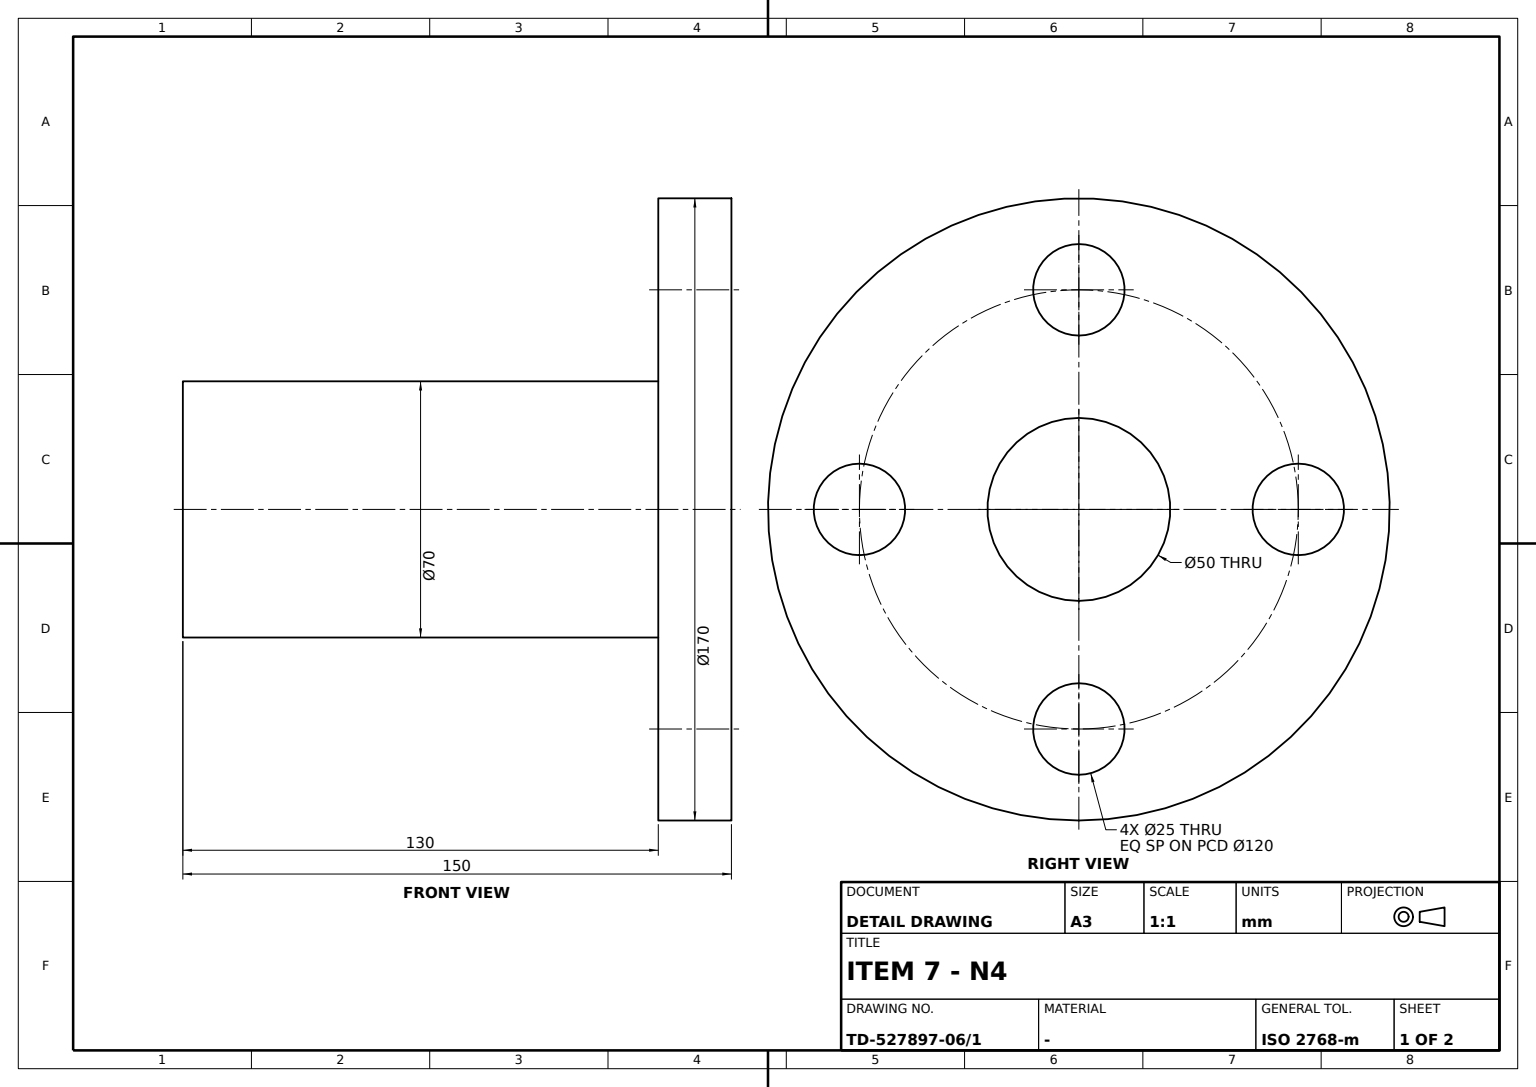
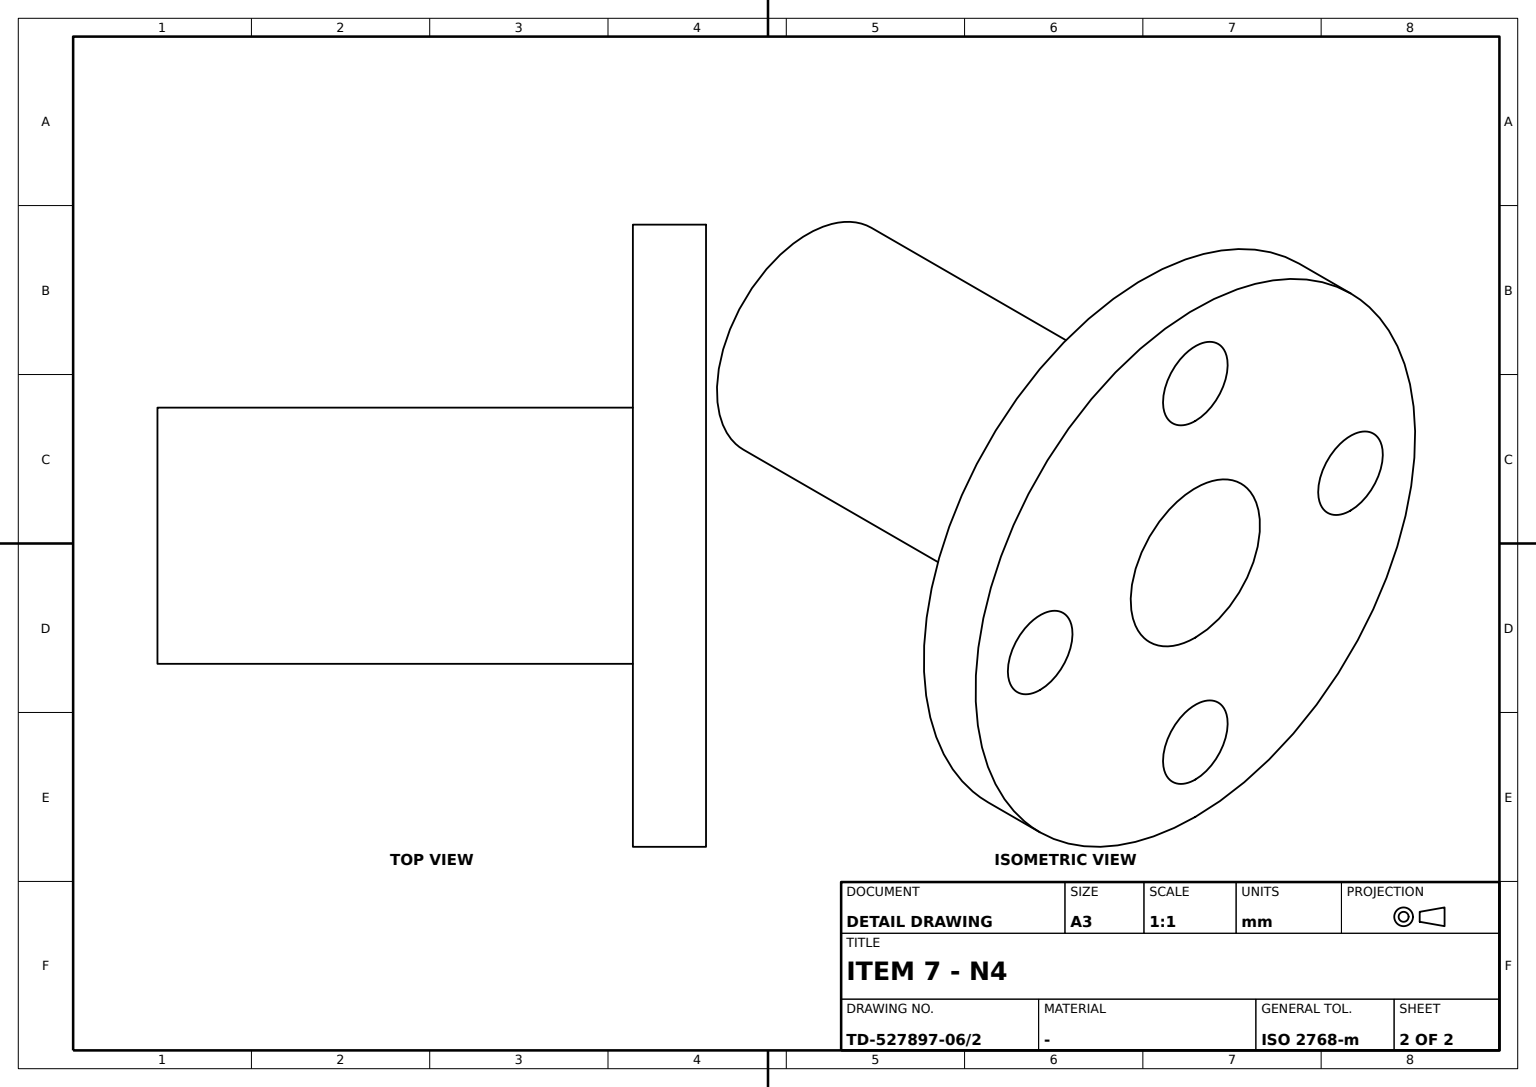
ISO-10303-21;
HEADER;
FILE_DESCRIPTION((''),'2;1');
FILE_NAME('','',(''),(''),'','','');
FILE_SCHEMA(('AUTOMOTIVE_DESIGN'));
ENDSEC;
DATA;
#1=APPLICATION_CONTEXT('');
#2=PRODUCT_CONTEXT('',#1,'mechanical');
#3=PRODUCT('','','',(#2));
#4=PRODUCT_DEFINITION_FORMATION('','',#3);
#5=PRODUCT_DEFINITION_CONTEXT('',#1,'design');
#6=PRODUCT_DEFINITION('','',#4,#5);
#7=PRODUCT_DEFINITION_SHAPE('','',#6);
#8=(LENGTH_UNIT()NAMED_UNIT(*)SI_UNIT(.MILLI.,.METRE.));
#9=(NAMED_UNIT(*)PLANE_ANGLE_UNIT()SI_UNIT($,.RADIAN.));
#10=(NAMED_UNIT(*)SI_UNIT($,.STERADIAN.)SOLID_ANGLE_UNIT());
#11=UNCERTAINTY_MEASURE_WITH_UNIT(LENGTH_MEASURE(0.005),#8,'distance_accuracy_value','');
#12=(GEOMETRIC_REPRESENTATION_CONTEXT(3)GLOBAL_UNCERTAINTY_ASSIGNED_CONTEXT((#11))GLOBAL_UNIT_ASSIGNED_CONTEXT((#8,#9,#10))REPRESENTATION_CONTEXT('',''));
#13=CARTESIAN_POINT('',(1202.5,1250.,2650.));
#14=VERTEX_POINT('',#13);
#15=CARTESIAN_POINT('',(1190.,1250.,2650.));
#16=DIRECTION('',(0.,0.,1.));
#17=DIRECTION('',(1.,0.,0.));
#18=AXIS2_PLACEMENT_3D('',#15,#16,#17);
#19=CIRCLE('',#18,12.5);
#20=EDGE_CURVE('',#14,#14,#19,.T.);
#21=ORIENTED_EDGE('',*,*,#20,.T.);
#22=EDGE_LOOP('',(#21));
#23=FACE_BOUND('',#22,.T.);
#24=CARTESIAN_POINT('',(1202.5,1250.,2630.));
#25=VERTEX_POINT('',#24);
#26=CARTESIAN_POINT('',(1190.,1250.,2630.));
#27=AXIS2_PLACEMENT_3D('',#26,#16,#17);
#28=CIRCLE('',#27,12.5);
#29=EDGE_CURVE('',#25,#25,#28,.T.);
#30=ORIENTED_EDGE('',*,*,#29,.F.);
#31=EDGE_LOOP('',(#30));
#32=FACE_BOUND('',#31,.T.);
#33=CARTESIAN_POINT('',(1190.,1250.,2640.));
#34=AXIS2_PLACEMENT_3D('',#33,#16,#17);
#35=CYLINDRICAL_SURFACE('',#34,12.5);
#36=ADVANCED_FACE('',(#23,#32),#35,.F.);
#37=CARTESIAN_POINT('',(1262.5,1190.,2630.));
#38=VERTEX_POINT('',#37);
#39=CARTESIAN_POINT('',(1250.,1190.,2630.));
#40=AXIS2_PLACEMENT_3D('',#39,#16,#17);
#41=CIRCLE('',#40,12.5);
#42=EDGE_CURVE('',#38,#38,#41,.T.);
#43=ORIENTED_EDGE('',*,*,#42,.T.);
#44=EDGE_LOOP('',(#43));
#45=FACE_BOUND('',#44,.T.);
#46=CARTESIAN_POINT('',(1335.,1250.,2630.));
#47=VERTEX_POINT('',#46);
#48=CARTESIAN_POINT('',(1250.,1250.,2630.));
#49=AXIS2_PLACEMENT_3D('',#48,#16,#17);
#50=CIRCLE('',#49,85.);
#51=EDGE_CURVE('',#47,#47,#50,.T.);
#52=ORIENTED_EDGE('',*,*,#51,.F.);
#53=EDGE_LOOP('',(#52));
#54=FACE_BOUND('',#53,.T.);
#55=CARTESIAN_POINT('',(1322.5,1250.,2630.));
#56=VERTEX_POINT('',#55);
#57=CARTESIAN_POINT('',(1310.,1250.,2630.));
#58=AXIS2_PLACEMENT_3D('',#57,#16,#17);
#59=CIRCLE('',#58,12.5);
#60=EDGE_CURVE('',#56,#56,#59,.T.);
#61=ORIENTED_EDGE('',*,*,#60,.T.);
#62=EDGE_LOOP('',(#61));
#63=FACE_BOUND('',#62,.T.);
#64=ORIENTED_EDGE('',*,*,#29,.T.);
#65=EDGE_LOOP('',(#64));
#66=FACE_BOUND('',#65,.T.);
#67=CARTESIAN_POINT('',(1262.5,1310.,2630.));
#68=VERTEX_POINT('',#67);
#69=CARTESIAN_POINT('',(1250.,1310.,2630.));
#70=AXIS2_PLACEMENT_3D('',#69,#16,#17);
#71=CIRCLE('',#70,12.5);
#72=EDGE_CURVE('',#68,#68,#71,.T.);
#73=ORIENTED_EDGE('',*,*,#72,.T.);
#74=EDGE_LOOP('',(#73));
#75=FACE_BOUND('',#74,.T.);
#76=CARTESIAN_POINT('',(1285.,1250.,2630.));
#77=VERTEX_POINT('',#76);
#78=CIRCLE('',#49,35.);
#79=EDGE_CURVE('',#77,#77,#78,.T.);
#80=ORIENTED_EDGE('',*,*,#79,.T.);
#81=EDGE_LOOP('',(#80));
#82=FACE_BOUND('',#81,.T.);
#83=CARTESIAN_POINT('',(0.,0.,2630.));
#84=AXIS2_PLACEMENT_3D('',#83,#16,#17);
#85=PLANE('',#84);
#86=ADVANCED_FACE('',(#45,#54,#63,#66,#75,#82),#85,.F.);
#87=ORIENTED_EDGE('',*,*,#51,.T.);
#88=EDGE_LOOP('',(#87));
#89=FACE_BOUND('',#88,.T.);
#90=CARTESIAN_POINT('',(1335.,1250.,2650.));
#91=VERTEX_POINT('',#90);
#92=CARTESIAN_POINT('',(1250.,1250.,2650.));
#93=AXIS2_PLACEMENT_3D('',#92,#16,#17);
#94=CIRCLE('',#93,85.);
#95=EDGE_CURVE('',#91,#91,#94,.T.);
#96=ORIENTED_EDGE('',*,*,#95,.F.);
#97=EDGE_LOOP('',(#96));
#98=FACE_BOUND('',#97,.T.);
#99=CARTESIAN_POINT('',(1250.,1250.,2640.));
#100=AXIS2_PLACEMENT_3D('',#99,#16,#17);
#101=CYLINDRICAL_SURFACE('',#100,85.);
#102=ADVANCED_FACE('',(#89,#98),#101,.T.);
#103=ORIENTED_EDGE('',*,*,#72,.F.);
#104=EDGE_LOOP('',(#103));
#105=FACE_BOUND('',#104,.T.);
#106=CARTESIAN_POINT('',(1262.5,1310.,2650.));
#107=VERTEX_POINT('',#106);
#108=CARTESIAN_POINT('',(1250.,1310.,2650.));
#109=AXIS2_PLACEMENT_3D('',#108,#16,#17);
#110=CIRCLE('',#109,12.5);
#111=EDGE_CURVE('',#107,#107,#110,.T.);
#112=ORIENTED_EDGE('',*,*,#111,.T.);
#113=EDGE_LOOP('',(#112));
#114=FACE_BOUND('',#113,.T.);
#115=CARTESIAN_POINT('',(1250.,1310.,2640.));
#116=AXIS2_PLACEMENT_3D('',#115,#16,#17);
#117=CYLINDRICAL_SURFACE('',#116,12.5);
#118=ADVANCED_FACE('',(#105,#114),#117,.F.);
#119=CARTESIAN_POINT('',(1275.,1250.,2500.));
#120=VERTEX_POINT('',#119);
#121=CARTESIAN_POINT('',(1250.,1250.,2500.));
#122=AXIS2_PLACEMENT_3D('',#121,#16,#17);
#123=CIRCLE('',#122,25.);
#124=EDGE_CURVE('',#120,#120,#123,.T.);
#125=ORIENTED_EDGE('',*,*,#124,.F.);
#126=EDGE_LOOP('',(#125));
#127=FACE_BOUND('',#126,.T.);
#128=CARTESIAN_POINT('',(1275.,1250.,2650.));
#129=VERTEX_POINT('',#128);
#130=CIRCLE('',#93,25.);
#131=EDGE_CURVE('',#129,#129,#130,.T.);
#132=ORIENTED_EDGE('',*,*,#131,.T.);
#133=EDGE_LOOP('',(#132));
#134=FACE_BOUND('',#133,.T.);
#135=CARTESIAN_POINT('',(1250.,1250.,2575.));
#136=AXIS2_PLACEMENT_3D('',#135,#16,#17);
#137=CYLINDRICAL_SURFACE('',#136,25.);
#138=ADVANCED_FACE('',(#127,#134),#137,.F.);
#139=ORIENTED_EDGE('',*,*,#79,.F.);
#140=EDGE_LOOP('',(#139));
#141=FACE_BOUND('',#140,.T.);
#142=CARTESIAN_POINT('',(1285.,1250.,2500.));
#143=VERTEX_POINT('',#142);
#144=CIRCLE('',#122,35.);
#145=EDGE_CURVE('',#143,#143,#144,.T.);
#146=ORIENTED_EDGE('',*,*,#145,.T.);
#147=EDGE_LOOP('',(#146));
#148=FACE_BOUND('',#147,.T.);
#149=CYLINDRICAL_SURFACE('',#136,35.);
#150=ADVANCED_FACE('',(#141,#148),#149,.T.);
#151=ORIENTED_EDGE('',*,*,#20,.F.);
#152=EDGE_LOOP('',(#151));
#153=FACE_BOUND('',#152,.T.);
#154=CARTESIAN_POINT('',(1262.5,1190.,2650.));
#155=VERTEX_POINT('',#154);
#156=CARTESIAN_POINT('',(1250.,1190.,2650.));
#157=AXIS2_PLACEMENT_3D('',#156,#16,#17);
#158=CIRCLE('',#157,12.5);
#159=EDGE_CURVE('',#155,#155,#158,.T.);
#160=ORIENTED_EDGE('',*,*,#159,.F.);
#161=EDGE_LOOP('',(#160));
#162=FACE_BOUND('',#161,.T.);
#163=ORIENTED_EDGE('',*,*,#131,.F.);
#164=EDGE_LOOP('',(#163));
#165=FACE_BOUND('',#164,.T.);
#166=ORIENTED_EDGE('',*,*,#111,.F.);
#167=EDGE_LOOP('',(#166));
#168=FACE_BOUND('',#167,.T.);
#169=CARTESIAN_POINT('',(1322.5,1250.,2650.));
#170=VERTEX_POINT('',#169);
#171=CARTESIAN_POINT('',(1310.,1250.,2650.));
#172=AXIS2_PLACEMENT_3D('',#171,#16,#17);
#173=CIRCLE('',#172,12.5);
#174=EDGE_CURVE('',#170,#170,#173,.T.);
#175=ORIENTED_EDGE('',*,*,#174,.F.);
#176=EDGE_LOOP('',(#175));
#177=FACE_BOUND('',#176,.T.);
#178=ORIENTED_EDGE('',*,*,#95,.T.);
#179=EDGE_LOOP('',(#178));
#180=FACE_BOUND('',#179,.T.);
#181=CARTESIAN_POINT('',(0.,0.,2650.));
#182=AXIS2_PLACEMENT_3D('',#181,#16,#17);
#183=PLANE('',#182);
#184=ADVANCED_FACE('',(#153,#162,#165,#168,#177,#180),#183,.T.);
#185=ORIENTED_EDGE('',*,*,#60,.F.);
#186=EDGE_LOOP('',(#185));
#187=FACE_BOUND('',#186,.T.);
#188=ORIENTED_EDGE('',*,*,#174,.T.);
#189=EDGE_LOOP('',(#188));
#190=FACE_BOUND('',#189,.T.);
#191=CARTESIAN_POINT('',(1310.,1250.,2640.));
#192=AXIS2_PLACEMENT_3D('',#191,#16,#17);
#193=CYLINDRICAL_SURFACE('',#192,12.5);
#194=ADVANCED_FACE('',(#187,#190),#193,.F.);
#195=ORIENTED_EDGE('',*,*,#42,.F.);
#196=EDGE_LOOP('',(#195));
#197=FACE_BOUND('',#196,.T.);
#198=ORIENTED_EDGE('',*,*,#159,.T.);
#199=EDGE_LOOP('',(#198));
#200=FACE_BOUND('',#199,.T.);
#201=CARTESIAN_POINT('',(1250.,1190.,2640.));
#202=AXIS2_PLACEMENT_3D('',#201,#16,#17);
#203=CYLINDRICAL_SURFACE('',#202,12.5);
#204=ADVANCED_FACE('',(#197,#200),#203,.F.);
#205=ORIENTED_EDGE('',*,*,#145,.F.);
#206=EDGE_LOOP('',(#205));
#207=FACE_BOUND('',#206,.T.);
#208=ORIENTED_EDGE('',*,*,#124,.T.);
#209=EDGE_LOOP('',(#208));
#210=FACE_BOUND('',#209,.T.);
#211=CARTESIAN_POINT('',(0.,0.,2500.));
#212=AXIS2_PLACEMENT_3D('',#211,#16,#17);
#213=PLANE('',#212);
#214=ADVANCED_FACE('',(#207,#210),#213,.F.);
#215=CLOSED_SHELL('',(#36,#86,#102,#118,#138,#150,#184,#194,#204,#214));
#216=MANIFOLD_SOLID_BREP('',#215);
#217=ADVANCED_BREP_SHAPE_REPRESENTATION('',(#216),#12);
#218=SHAPE_DEFINITION_REPRESENTATION(#7,#217);
ENDSEC;
END-ISO-10303-21;
